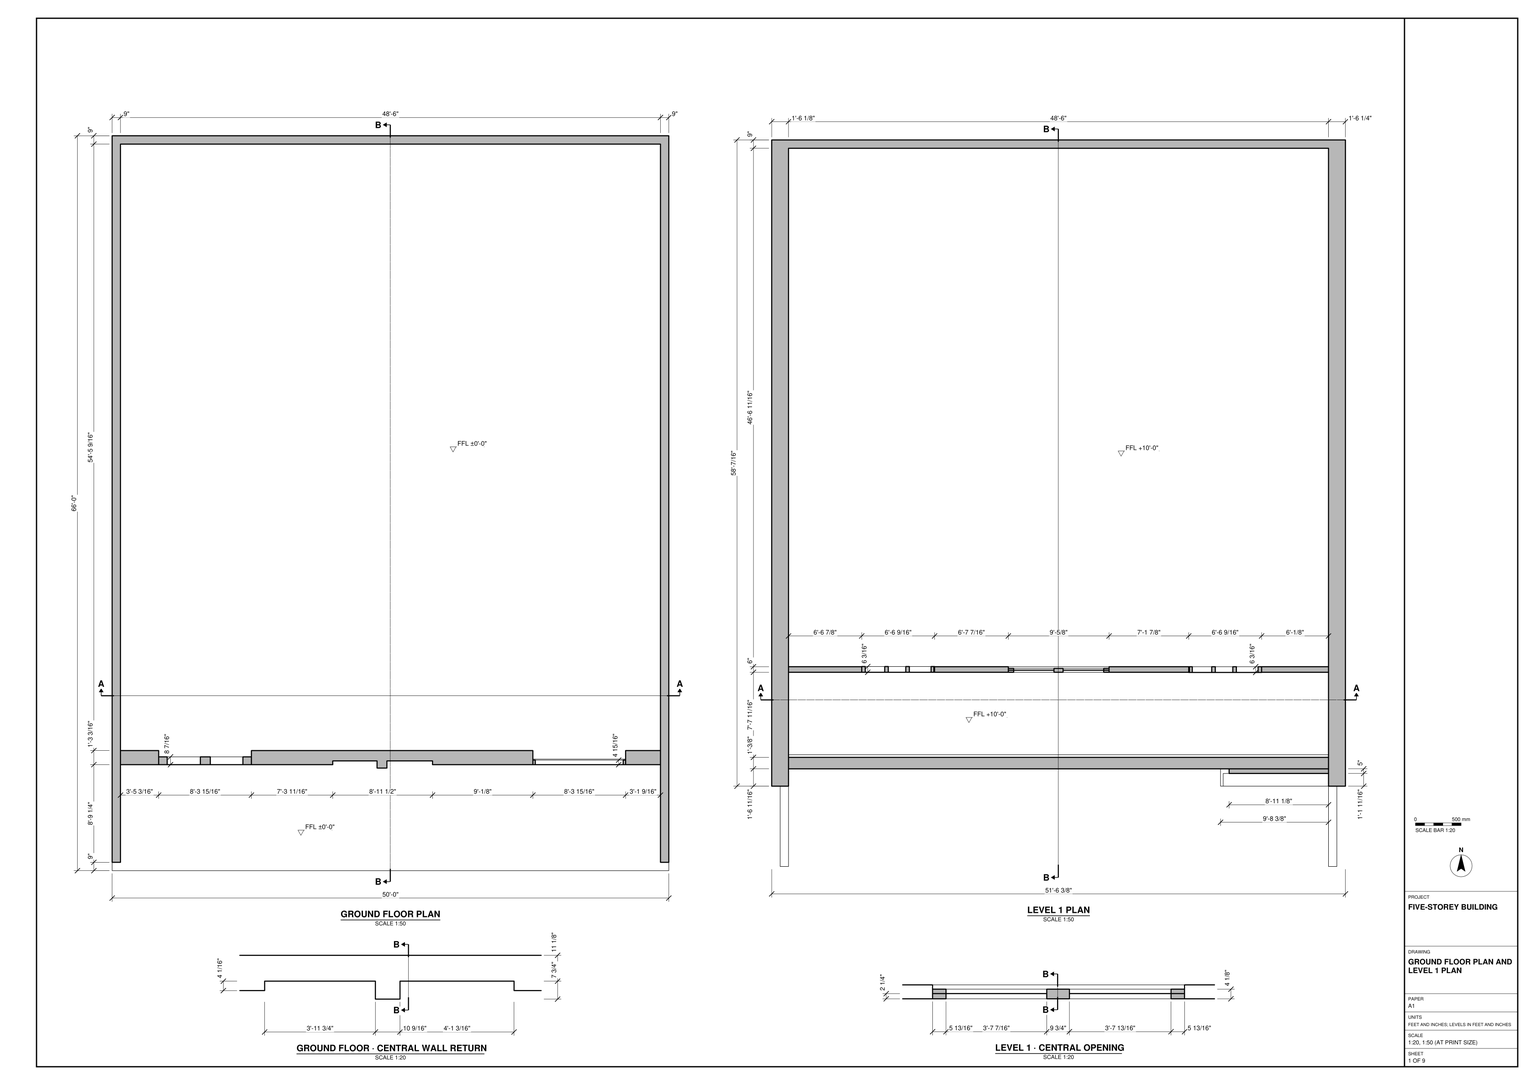
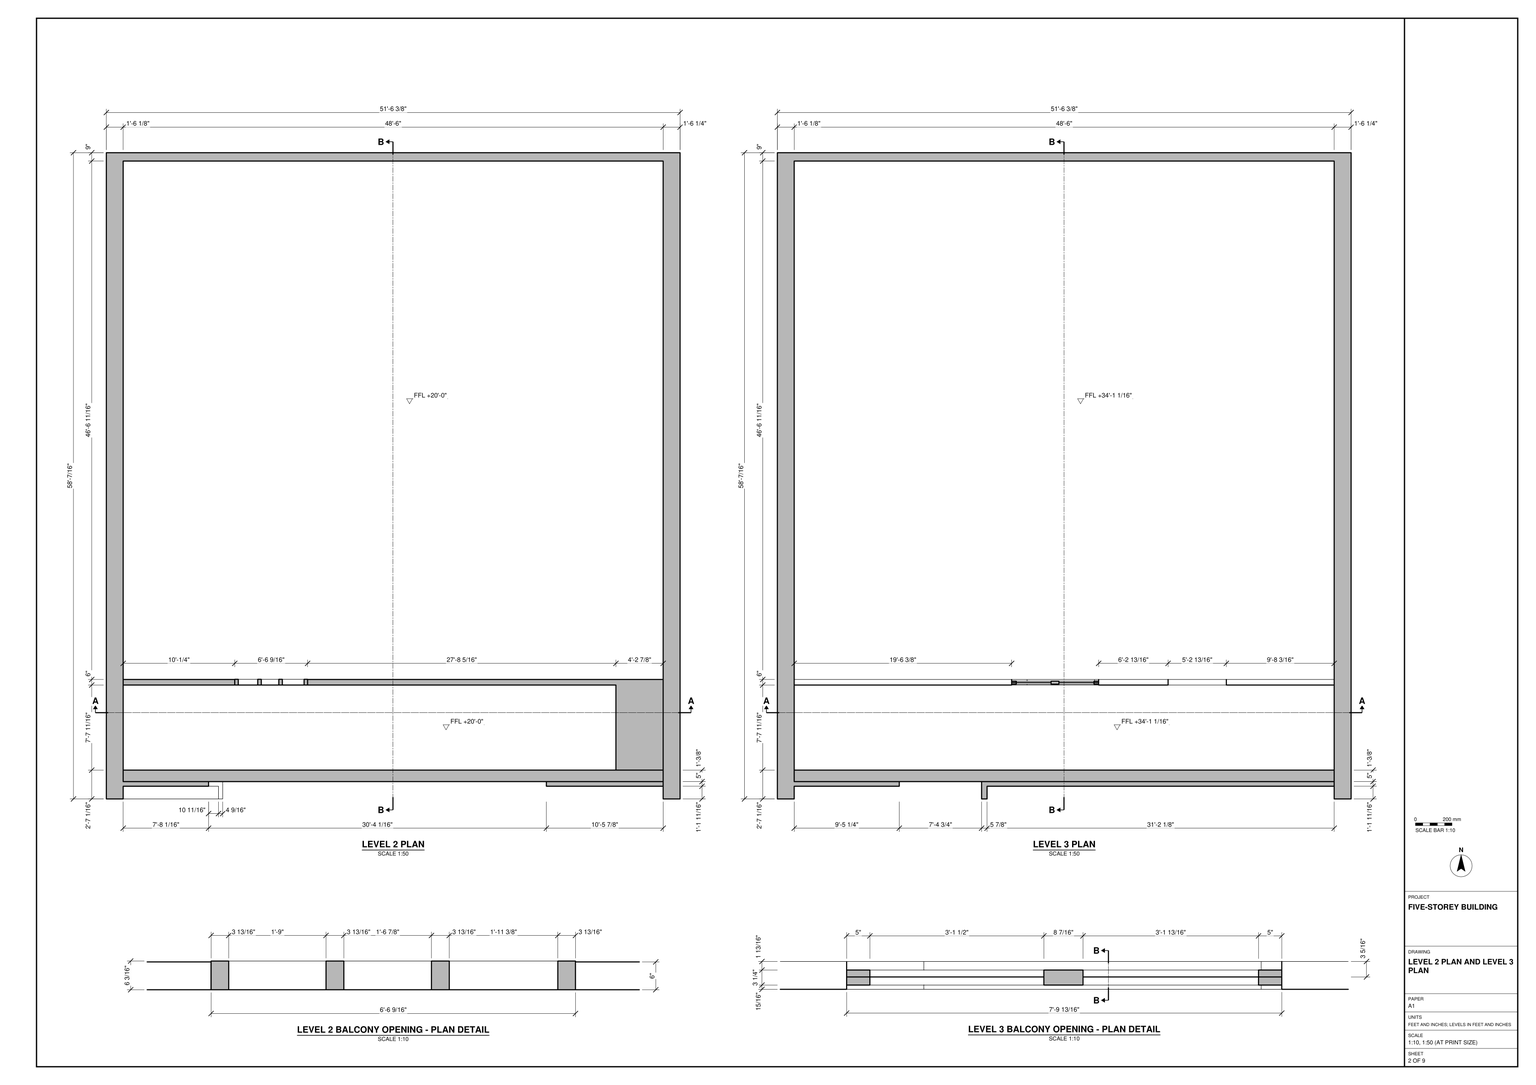
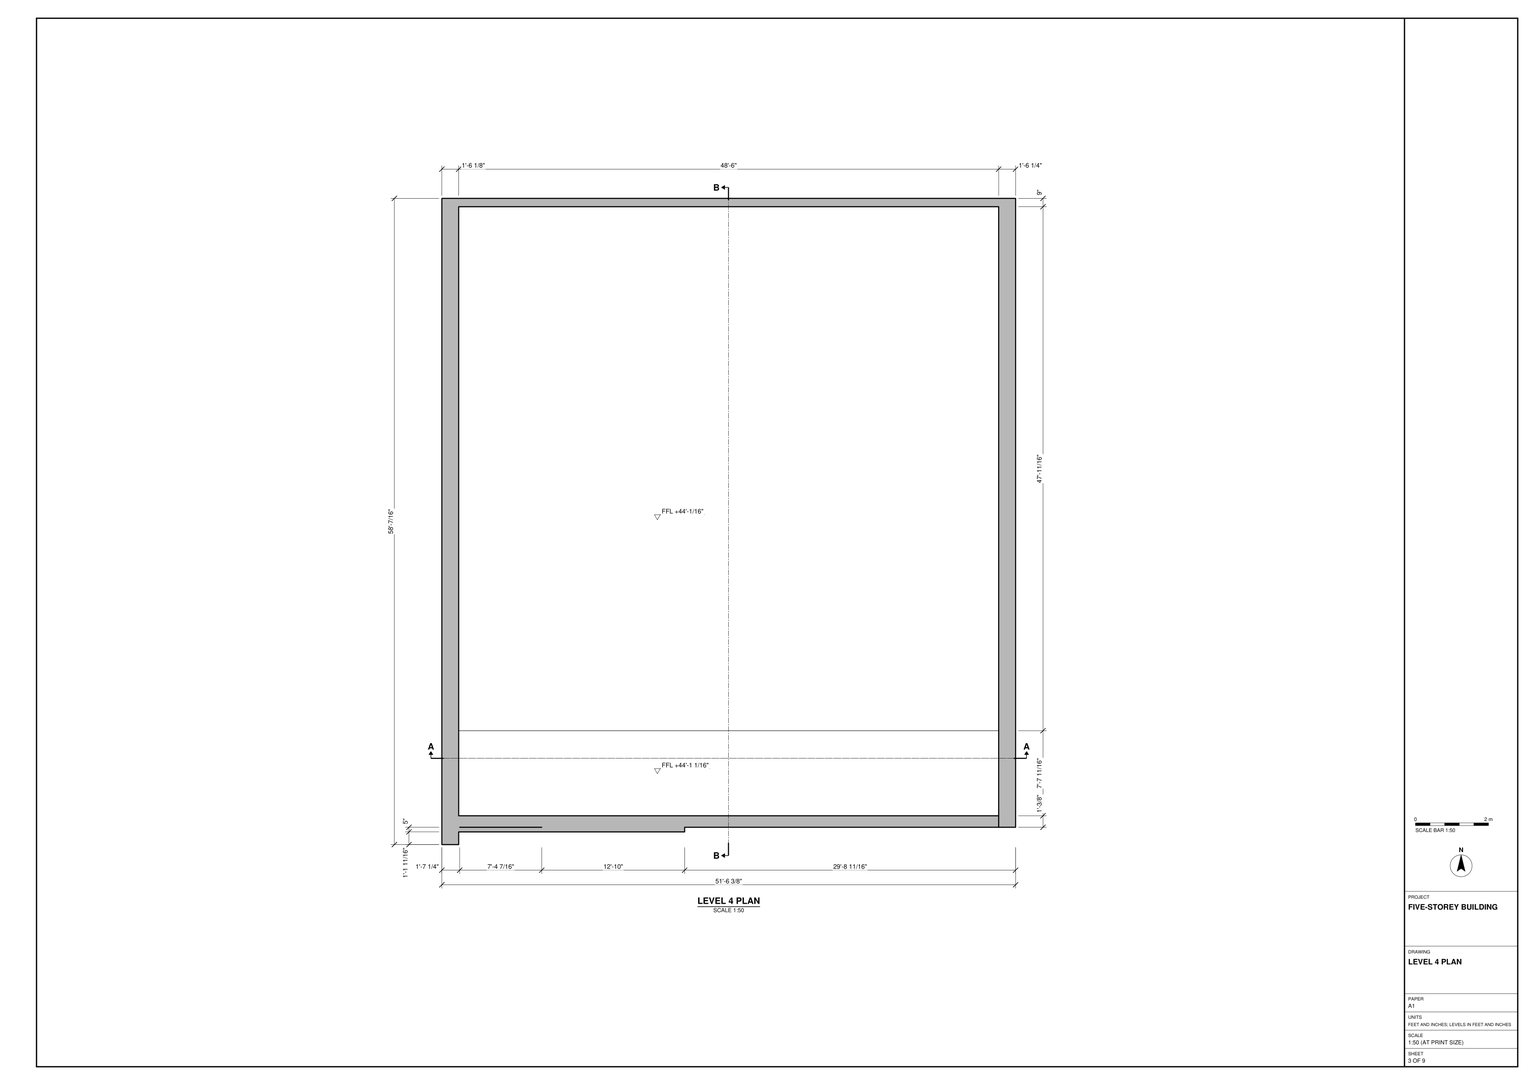
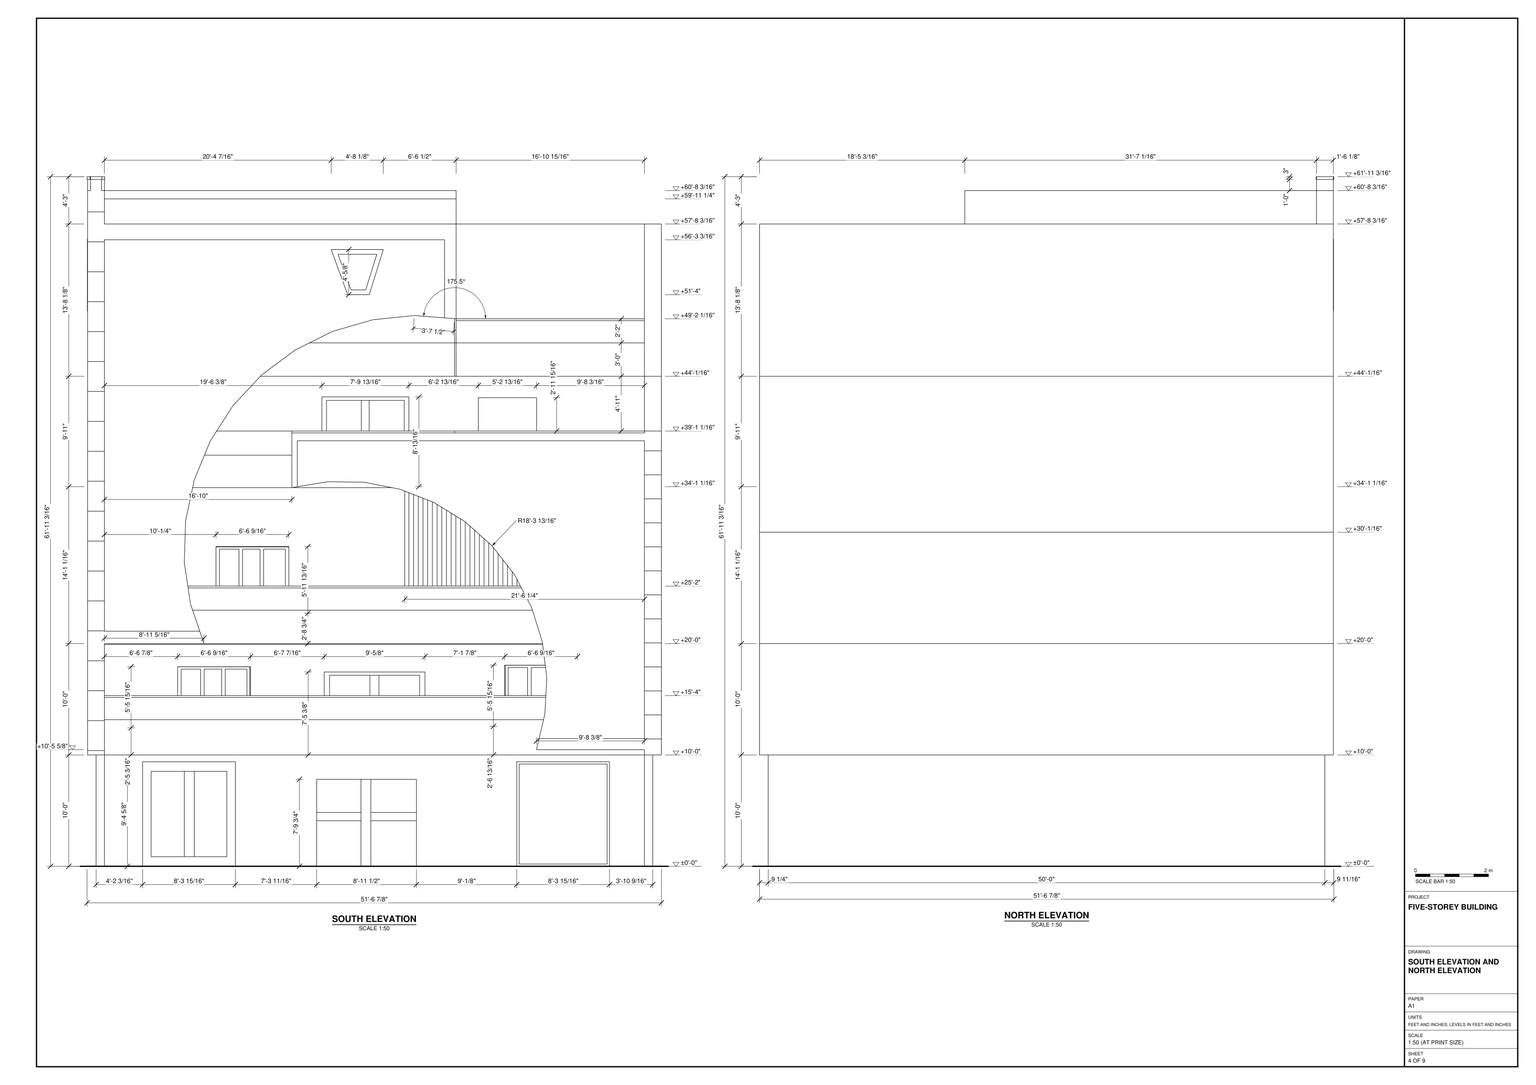
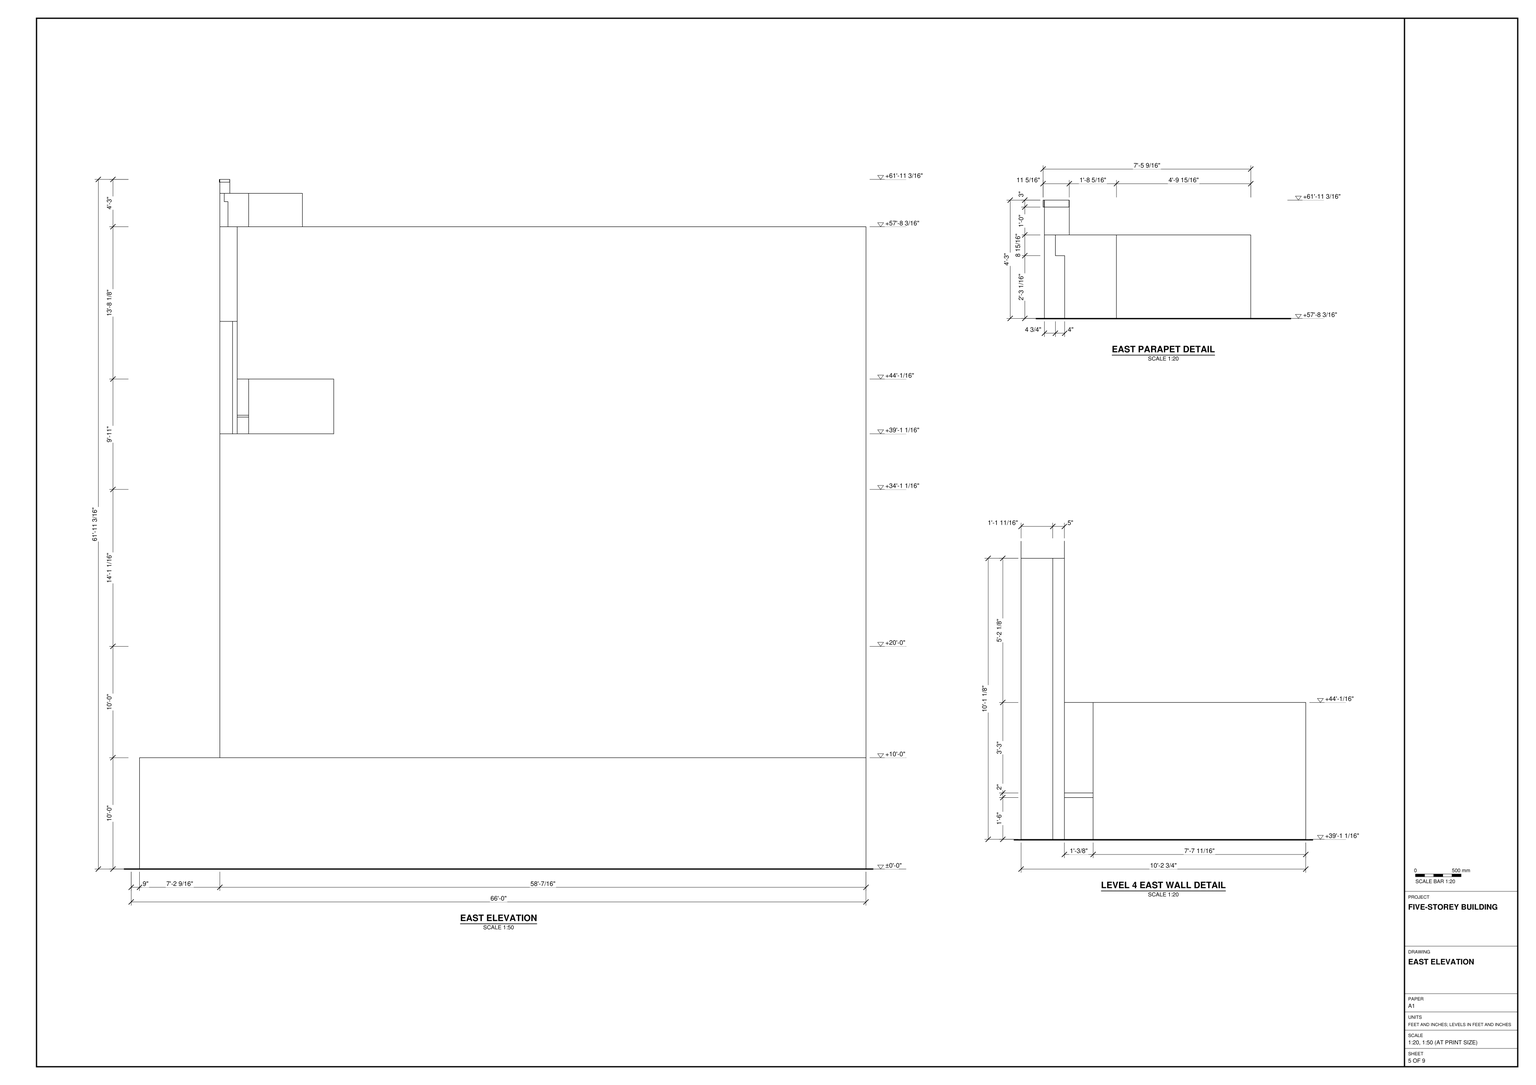
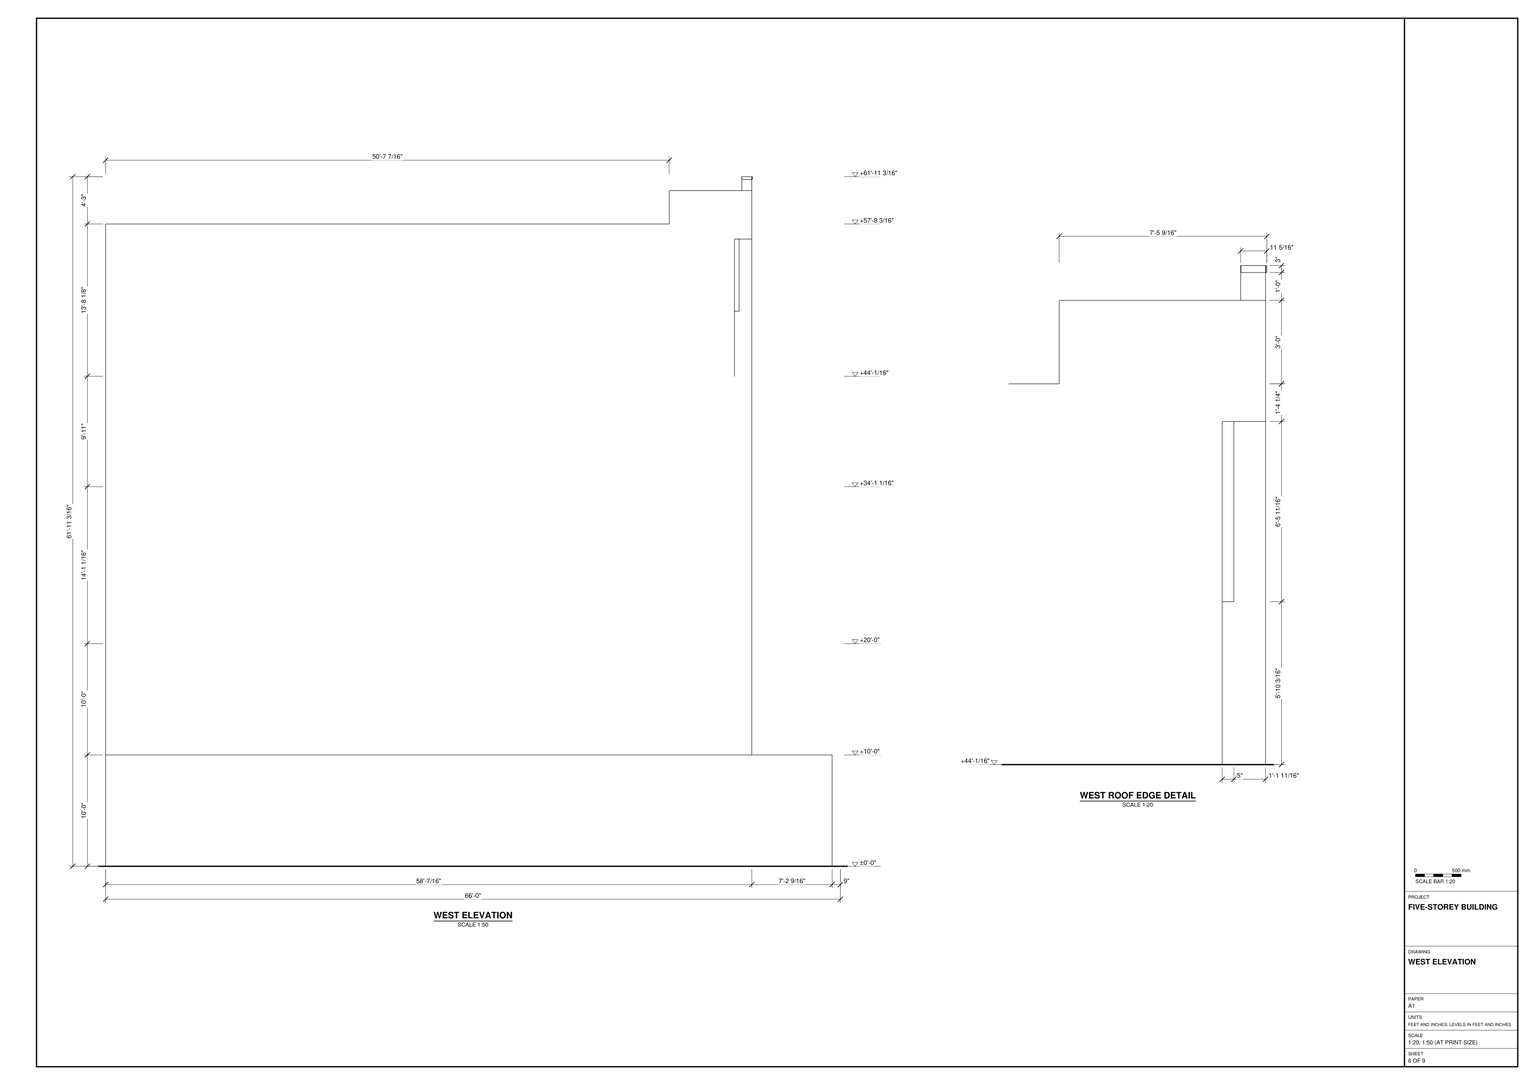
Build the five-storey building in SketchUp from task_files/diagram_01.pdf. Work in feet and inches. The overall width is 51'-6 15/16", the front-to-back depth is 66'-0", and the height is 61'-11 3/16". Set the finished floor levels to ±0'-0", +10'-0", +20'-0", +34'-1 1/16", and +44'-1/16".

Start with the deeper ground-floor slab. Model the side walls extending past the recessed front wall, including the openings on either side of its stepped central return. Use the wall thicknesses drawn at each level: the upper side walls are thicker than those on the ground floor. Keep the large floor areas open as drawn. Form the front balconies on Levels 1 through 3, following each plan for the slab edge, wall returns and framed openings rather than copying one frontage to every level. Follow the Level 4 plan for the stepped front edge and use the sections and elevations to complete the roof and facade above it.

Keep walls, slabs and roof in separate groups or components. Keep each furniture or joinery piece shown separate as well, and use components for repeated parts. Any decor or loose items shown may be represented by suitable library components. Save one SketchUp model as output_files/five_storey_building_with_recessed_front_balconies.skp.

# SketchUp Ruby script. Lengths in inches.
U = 1.inch
M = Sketchup.active_model
def pt(a) = Geom::Point3d.new(a.map { |v| v * U })
def face(e, loops, mat)
  f = e.add_face(loops[0].map { |a| pt(a) })
  loops[1..].each { |l| e.add_face(l.map { |a| pt(a) }).erase! }
  f.material = f.back_material = mat if mat
  f
end
# faces: each face lists its corners as indices into pts; further lists are holes
def faces(e, pts, list, mat = nil) = list.each { |f| face(e, (f[0].is_a?(Array) ? f : [f]).map { |l| l.map { |i| pts[i] } }, mat) }
# xy, xz, yz: faces in a plane at the given z, y or x. An outline is a flat list of corners, or four numbers for a rectangle; further outlines are holes
def ring(l) = l.size == 4 ? [[l[0], l[1]], [l[2], l[1]], [l[2], l[3]], [l[0], l[3]]] : l.each_slice(2).to_a
def flat(e, list, mat, &to3) = list.each { |f| face(e, (f[0].is_a?(Array) ? f : [f]).map { |l| ring(l).map { |u, v| to3.(u, v) } }, mat) }
def xy(e, z, list, mat = nil) = flat(e, list, mat) { |x, y| [x, y, z] }
def xz(e, y, list, mat = nil) = flat(e, list, mat) { |x, z| [x, y, z] }
def yz(e, x, list, mat = nil) = flat(e, list, mat) { |y, z| [x, y, z] }
def lines(e, pts, list) = list.each { |a, b| e.add_line(pt(pts[a]), pt(pts[b])) }
# prism: a flat outline (further loops are holes) pulled along v
def prism(e, loops, v, mat = nil)
  f = face(e, loops, mat); d = Geom::Vector3d.new(v.map { |x| x * U })
  f.pushpull(f.normal.samedirection?(d) ? d.length : -d.length)
end
def box(e, o, s, mat = nil) = prism(e, [[o, [o[0] + s[0], o[1], o[2]], [o[0] + s[0], o[1] + s[1], o[2]], [o[0], o[1] + s[1], o[2]]]], [0, 0, s[2]], mat)
def at(x, y, z, deg = 0) = Geom::Transformation.translation(pt([x, y, z])) * Geom::Transformation.rotation(ORIGIN, Z_AXIS, deg.degrees)
def axes(o, x, y, z) = Geom::Transformation.new([*x, 0, *y, 0, *z, 0, *pt(o).to_a, 1])
def part(name) = M.definitions.add(name)
# library, detail: a bought-in or finely detailed component or shape, given as its bounding box
def library(name, o, s) = part(name).tap { |d| box(d.entities, o, s) }
def detail(e, o, s) = box(e.add_group.entities, o, s)
def put(e, d, t, mat = nil) = e.add_instance(d, t).tap { |i| i.material = mat if mat }
def group(e, t, mat = nil) = e.add_group.tap { |g| g.transformation = t; g.material = mat if mat }.entities
root = M.entities
M.materials.add("[Aluminum]").color = [179, 179, 179]
M.materials.add("[Blinds Roman Hobbled Blue]").color = [81, 82, 87]
M.materials.add("[Blinds Wood Light]").color = [155, 100, 14]
M.materials.add("[Color D06]").color = [204, 153, 0]
M.materials.add("[Color M00]").color = [255, 255, 255]
M.materials.add("[Metal Silver]").color = [234, 233, 238]
M.materials.add("[Polished Concrete Old]").color = [229, 229, 229]
M.materials.add("[Translucent Glass Gray]").color = [128, 128, 128]
M.materials["[Translucent Glass Gray]"].alpha = 0.5
M.materials.add("[Wood Bamboo]").color = [177, 105, 43]
M.materials.add("[Wood Floor]").color = [155, 105, 61]
c1 = part("Group\#3")
xy(c1.entities,0,[[0,0,110.8125,6]])
xy(c1.entities,5.36,[[5.36,0,34.95,6],[40.375,0,67.02,6],[72.4375,0,105.45,6]])
xy(c1.entities,134.51,[[5.36,0,34.95,6],[40.375,0,67.02,6],[72.4375,0,105.45,6]])
xy(c1.entities,139.875,[[0,0,110.8125,6]])
xz(c1.entities,0,[[[0,0,110.8125,139.875],[72.4375,5.36,105.45,134.51],[5.36,5.36,34.95,134.51],[40.375,5.36,67.02,134.51]]])
xz(c1.entities,0,[[5.36,5.36,34.95,134.51],[40.375,5.36,67.02,134.51],[72.4375,5.36,105.45,134.51]],"[Translucent Glass Gray]")
xz(c1.entities,6,[[[0,0,110.8125,139.875],[72.4375,5.36,105.45,134.51],[5.36,5.36,34.95,134.51],[40.375,5.36,67.02,134.51]]])
yz(c1.entities,0,[[0,0,6,139.875]])
yz(c1.entities,5.36,[[0,5.36,6,134.51]])
yz(c1.entities,34.95,[[0,5.36,6,134.51]])
yz(c1.entities,40.375,[[0,5.36,6,134.51]])
yz(c1.entities,67.02,[[0,5.36,6,134.51]])
yz(c1.entities,72.4375,[[0,5.36,6,134.51]])
yz(c1.entities,105.45,[[0,5.36,6,134.51]])
yz(c1.entities,110.8125,[[0,0,6,139.875]])
c2 = part("Group\#4")
xy(c2.entities,0,[[0,0,126.375,7],[0,7,126.375,13]])
xy(c2.entities,6.76,[[57.28,0,68.66,7],[6.76,7,57.28,13],[57.28,7,68.66,13],[68.66,7,119.62,13]])
xy(c2.entities,6.76,[[6.76,0,57.28,7],[68.66,0,119.62,7]],"[Wood Floor]")
xy(c2.entities,165.31,[[57.28,0,68.66,7],[6.76,7,57.28,13],[57.28,7,68.66,13],[68.66,7,119.62,13]])
xy(c2.entities,165.31,[[6.76,0,57.28,7],[68.66,0,119.62,7]],"[Wood Floor]")
xy(c2.entities,172.0625,[[0,0,126.375,7],[0,7,126.375,13]])
xz(c2.entities,0,[[57.28,6.76,68.66,165.31]])
xz(c2.entities,0,[[[0,0,126.375,172.0625],[6.76,6.76,119.62,165.31]]],"[Wood Floor]")
xz(c2.entities,7,[[[0,0,126.375,172.0625],[6.76,6.76,119.62,165.31]]])
xz(c2.entities,7,[[6.76,6.76,57.28,165.31],[68.66,6.76,119.62,165.31]],"[Wood Floor]")
xz(c2.entities,13,[[[0,0,126.375,172.0625],[6.76,6.76,119.62,165.31]],[57.28,6.76,68.66,165.31]])
yz(c2.entities,0,[[0,0,7,172.0625],[7,0,13,172.0625]])
yz(c2.entities,6.76,[[7,6.76,13,165.31]])
yz(c2.entities,6.76,[[0,6.76,7,165.31]],"[Wood Floor]")
yz(c2.entities,57.28,[[0,6.76,7,165.31],[7,6.76,13,165.31]])
yz(c2.entities,68.66,[[0,6.76,7,165.31],[7,6.76,13,165.31]])
yz(c2.entities,119.62,[[7,6.76,13,165.31]])
yz(c2.entities,119.62,[[0,6.76,7,165.31]],"[Wood Floor]")
yz(c2.entities,126.375,[[0,0,7,172.0625],[7,0,13,172.0625]])
xy(root,0,[[9.66,0,609.66,0,609.66,9,600.66,9,600.66,114.25,563.09,114.25,563.09,120.25,463.14,120.25,463.14,114.25,354.98,114.25,354.98,118.3125,305.81,118.3125,305.81,110.5625,295.19,110.5625,295.19,118.3125,247.45,118.3125,247.45,114.25,159.78,114.25,159.78,120.25,59.83,120.25,59.83,114.25,18.66,114.25,18.66,9,9.66,9],[9.66,9,9.66,792,609.66,792,609.66,9,600.66,9,600.66,783,18.66,783,18.66,9],[295.19,110.5625,295.19,118.3125,247.45,118.3125,247.45,114.25,159.78,114.25,159.78,129.4375,463.14,129.4375,463.14,114.25,354.98,114.25,354.98,118.3125,305.81,118.3125,305.81,110.5625],[18.66,114.25,59.83,129.4375],[563.09,114.25,600.66,129.4375],
  [59.83,120.25,159.78,120.25,159.78,129.4375,463.14,129.4375,463.14,120.25,563.09,120.25,563.09,129.4375,600.66,129.4375,600.66,783,18.66,783,18.66,129.4375,59.83,129.4375]])
xy(root,93.73,[[295.19,110.5625,305.81,114.25]])
xy(root,93.73,[[247.45,114.25,295.19,118.3125],[305.81,114.25,354.98,118.3125]],"[Blinds Wood Light]")
xy(root,112.63,[[59.83,114.25,159.78,129.4375],[463.14,114.25,563.09,129.4375]])
xy(root,120,[[9.66,9,18.66,95.5625],[600.66,9,609.66,95.5625],[0.54,95.5625,9.66,792],[609.66,95.5625,618.91,792],[18.66,114.25,600.66,126.625],
  [18.66,126.625,600.66,129.4375],[18.66,129.4375,600.66,129.4375,600.66,218.3125,364.17,218.3125,364.17,224.3125,255.54,224.3125,255.54,218.3125,18.66,218.3125],[18.66,224.3125,600.66,783]])
xy(root,125.65,[[484.29,95.5625,600.66,114.25]],"[Polished Concrete Old]")
xy(root,137.67,[[487.14,95.5625,600.66,109.25]],"[Polished Concrete Old]")
xy(root,149.16,[[97.56,218.3125,175.31,224.3125]])
xy(root,150.8125,[[450.8125,218.3125,528.5625,224.3125]])
xy(root,158,[[18.66,114.25,600.66,126.625]])
xy(root,182,[[18.66,114.25,600.66,126.625]])
xy(root,184,[[18.66,114.25,600.66,126.625]],"[Metal Silver]")
xy(root,209.375,[[255.54,218.3125,364.17,224.3125]])
xy(root,214.97,[[97.56,218.3125,175.31,224.3125]])
xy(root,216.625,[[450.8125,218.3125,528.5625,224.3125]])
xy(root,239,[[18.66,126.625,600.66,218.3125],[18.66,224.3125,600.66,783]])
xy(root,240,[[18.66,95.5625,125.96,114.25],[18.66,114.25,600.66,126.625],[18.66,126.625,549.76,218.3125],[549.76,126.625,600.66,218.3125],[18.66,224.3125,600.66,783]])
xy(root,253.36,[[18.66,95.5625,121.41,109.25]])
xy(root,272.73,[[138.9,218.3125,217.46,224.3125]])
xy(root,276,[[18.66,114.25,600.66,126.625]])
xy(root,300,[[18.66,114.25,600.66,126.625]])
xy(root,302,[[18.66,114.25,600.66,126.625]],"[Metal Silver]")
xy(root,344.17,[[138.9,218.3125,217.46,224.3125]])
xy(root,408.0625,[[18.66,114.25,600.66,126.625],[18.66,126.625,549.76,218.3125],[549.76,126.625,600.66,218.3125],[18.66,218.3125,600.66,224.3125],[18.66,224.3125,600.66,783]])
xy(root,409.0625,[[18.66,126.625,600.66,218.3125],[253.02,218.3125,269.66,224.3125],[269.66,218.3125,342.38,224.3125],[342.38,218.3125,346.82,224.3125],[18.66,224.3125,600.66,783]])
xy(root,442.21,[[421.65,218.3125,484.46,224.3125]])
xy(root,443.0625,[[18.66,114.25,600.66,126.625]])
xy(root,458.58,[[226.55,95.5625,600.66,109.25]],"[Polished Concrete Old]")
xy(root,467.0625,[[220.66,95.5625,600.66,109.25],[220.66,109.25,600.66,114.25]],"[Polished Concrete Old]")
xy(root,469.0625,[[600.66,95.5625,618.91,218.3125]])
xy(root,469.0625,[[18.66,114.25,600.66,126.625]],"[Metal Silver]")
xy(root,505.02,[[421.65,218.3125,484.46,224.3125]])
xy(root,505.86,[[253.02,218.3125,346.82,224.3125]])
xy(root,528.0625,[[18.66,114.25,600.66,126.625],[18.66,126.625,600.66,218.3125],[18.66,218.3125,600.66,783]])
xy(root,528.0625,[[600.66,114.25,618.91,218.3125]],"[Polished Concrete Old]")
xy(root,529.0625,[[18.66,126.625,600.66,218.3125]])
xy(root,564.0625,[[18.66,114.25,600.66,126.625]])
xy(root,590.0625,[[397.73,114.25,397.75,126.625],[397.75,114.25,600.66,126.625]],"[Metal Silver]")
xy(root,590.19,[[396.08,95.5625,397.73,114.25]])
xy(root,598.28,[[0.27,109.25,0.54,114.25]])
xy(root,616.02,[[280.84,95.5625,304.09,109.25]],"[Color M00]")
xy(root,621.15,[[284.43,95.5625,300.3125,109.25]],"[Color M00]")
xy(root,659.53,[[270.42,95.5625,312.24,109.25]],"[Color M00]")
xy(root,664.66,[[263.09,95.5625,319.21,109.25]],"[Color M00]")
xy(root,675.1875,[[18.66,95.5625,385.27,109.25]])
xy(root,675.97,[[0.27,109.25,0.54,114.25]])
xy(root,692.1875,[[18.66,95.5625,397.73,104.3125],[600.66,114.25,618.91,114.25,618.91,792,0.54,792,0.54,184.54,18.66,184.54,18.66,783,600.66,783]])
xy(root,719.25,[[18.66,100.3125,397.73,104.3125]],"[Color M00]")
xy(root,728.1875,[[0.54,95.5625,3.7,95.5625,0.54,106.31],[15.52,95.5625,18.66,95.5625,18.66,106.31],[18.66,100.3125,397.73,126.625],[0.54,106.31,18.66,184.54]])
xy(root,740.1875,[[3.2,95,3.2,95.42,3.7,95.5625,3.7,95],[3.7,95,3.7,95.5625,15.52,95.5625,15.94,95.44,15.96,95.5,15.96,95],[3.16,95.4,0,106.15,0.54,106.31,3.7,95.5625,3.2,95.5625,3.2,95.42],[3.2,95.42,3.2,95.5625,3.7,95.5625],[15.94,95.44,15.52,95.5625,15.96,95.5625,15.96,95.5],
  [15.96,95.5,15.96,95.5625,15.52,95.5625,18.66,106.31,19.08,106.18],[[3.7,95.5625,0.54,106.31,18.66,106.31,15.52,95.5625],[4.6875,96.88,14.54,96.88,16.9,104.99,2.3,104.99]],[4.6875,96.88,14.54,96.88,16.9,104.99,2.3,104.99]])
xy(root,743.1875,[[3.2,95,3.7,95,3.7,95.5625,0.54,106.31,0,106.15,3.16,95.4,3.2,95.42],[[3.7,95,15.96,95,15.96,95.5,19.08,106.18,18.66,106.31,0.54,106.31,3.7,95.5625],[4.6875,96.88,2.3,104.99,16.9,104.99,14.54,96.88]]])
xz(root,9,[[9.66,0,18.66,120],[600.66,0,609.66,120]])
xz(root,95,[[3.2,740.1875,3.7,743.1875],[3.7,740.1875,15.96,743.1875]])
xz(root,95.5625,[[0.54,120,18.66,124.73],[600.66,120,618.91,120,618.91,163.13,600.66,163.13,600.66,137.67,487.14,137.67,484.29,125.65,600.66,125.65],[0.54,124.73,18.66,156.98],[0.54,156.98,18.66,189.23],[600.66,163.13,618.91,189],
  [600.66,189,618.91,214.88],[0.54,189.23,18.66,221.48],[600.66,214.88,618.91,240.75],[0.54,221.48,18.66,221.48,18.66,240,125.96,240,121.41,253.36,18.66,253.36,18.66,253.73,0.54,253.73],[600.66,240.75,618.91,266.63],
  [0.54,253.73,18.66,285.98],[600.66,266.63,618.91,292.5],[0.54,285.98,18.66,318.23],[600.66,292.5,618.91,318.38],[0.54,318.23,18.66,350.48],
  [600.66,318.38,618.91,344.25],[600.66,344.25,618.91,370.13],[0.54,350.48,18.66,382.73],[600.66,370.13,618.91,396],[0.54,382.73,18.66,414.98],
  [600.66,396,618.91,421.88],[220.66,408.0625,226.55,409.04,226.55,458.58,600.66,458.58,600.66,447.75,618.91,447.75,618.91,469.0625,600.66,469.0625,600.66,467.0625,220.66,467.0625],[0.54,414.98,18.66,447.23],[600.66,421.88,618.91,447.75],[0.54,447.23,18.66,479.48],
  [0.54,479.48,18.66,511.73],[0.54,511.73,18.66,543.98],[0.54,543.98,18.66,576.23],[0.54,576.23,18.66,608.48],[396.08,590.19,397.73,590.19,397.73,692.1875,18.66,692.1875,18.66,705.23,0.54,705.23,0.54,672.98,18.66,672.98,18.66,675.1875,385.27,675.1875,385.27,591.03],
  [0.54,608.48,18.66,640.73],[0.54,640.73,18.66,672.98],[0.54,705.23,18.66,705.23,18.66,728.1875,15.52,728.1875,15.52,740.1875,3.7,740.1875,3.7,728.1875,0.54,728.1875]])
xz(root,95.5625,[[[280.84,616.02,304.09,616.02,319.21,664.66,263.09,664.66],[284.43,621.15,270.42,659.53,312.24,659.53,300.3125,621.15]]],"[Color M00]")
xz(root,96.88,[[4.6875,740.1875,14.54,743.1875]])
xz(root,100.3125,[[18.66,719.25,397.73,728.1875]],"[Color M00]")
xz(root,104.3125,[[18.66,692.1875,397.73,719.25]],"[Color M00]")
xz(root,104.99,[[2.3,740.1875,16.9,743.1875]])
xz(root,106.31,[[0.54,728.1875,18.66,740.1875],[0.54,740.1875,18.66,743.1875]])
xz(root,109.25,[[0.27,598.28,0.54,675.97]])
xz(root,109.25,[[284.43,621.15,300.3125,621.15,312.24,659.53,270.42,659.53]],"[Color M00]")
xz(root,109.25,[[487.14,137.67,600.66,137.67,600.66,458.58,226.55,458.58,226.55,409.04,259.41,414.48,298.67,413.91,337.21,406.35,373.79,392.0625,407.24,371.49,436.5,345.29,460.62,314.3,478.85,279.52,490.59,242.04,495.48,203.08,493.36,163.86],[[18.66,253.36,121.41,253.36,111.41,282.72,104.73,327.36,106.14,372.47,115.59,416.6,132.77,458.33,157.13,496.32,187.9,529.34,224.07,556.34,264.48,576.43,307.83,588.97,352.73,593.57,385.27,591.03,385.27,675.1875,18.66,675.1875],[280.84,616.02,263.09,664.66,319.21,664.66,304.09,616.02]]],"[Wood Bamboo]")
xz(root,110.5625,[[295.19,0,305.81,93.73]])
xz(root,114.25,[[18.66,0,59.83,0,59.83,112.63,159.78,112.63,159.78,0,247.45,0,247.45,93.73,354.98,93.73,354.98,0,463.14,0,463.14,112.63,563.09,112.63,563.09,0,600.66,0,600.66,120,18.66,120],[18.66,240,19.77,276],[19.77,240,108.21,276],[108.21,240,108.21,276,113.7,276,125.96,240],[490.85,240,490.59,242.04,479.95,276,600.66,276,600.66,240],
  [18.66,276,18.66,564.0625,19.77,564.0625,19.77,598.28,108.21,598.28,108.21,528.0625,19.77,528.0625,19.77,469.0625,108.21,469.0625,108.21,467.0625,19.77,467.0625,19.77,302,108.21,302,108.21,276],[18.66,276,19.77,300],[108.21,276,108.21,300,108.83,300,111.41,282.72,113.7,276],[18.66,302,19.77,408.0625],[19.77,302,19.77,408.0625,113.76,408.0625,106.14,372.47,104.73,327.36,108.53,302],
  [19.77,443.0625,19.77,467.0625,138.37,467.0625,132.77,458.33,126.48,443.0625],[220.66,443.0625,600.66,467.0625],[220.66,467.0625,396.08,469.0625],[396.08,467.0625,600.66,469.0625],[18.66,469.0625,19.77,528.0625],
  [108.21,528.0625,108.21,564.0625,239.61,564.0625,224.07,556.34,187.9,529.34,186.7,528.0625],[186.7,528.0625,396.08,528.0625,396.08,564.0625,239.61,564.0625,224.07,556.34,187.9,529.34],[19.77,564.0625,108.21,598.28],[239.61,564.0625,396.08,564.0625,396.08,590.19,352.73,593.57,307.83,588.97,264.48,576.43],[396.08,564.0625,397.75,564.0625,397.75,590.0625,397.73,590.0625,397.73,590.19,396.08,590.19],
  [0.27,598.28,0.54,675.97]])
xz(root,114.25,[[18.66,182,494.34,182,494.45,184,18.66,184],[18.66,300,19.77,302],[19.77,300,108.21,302],[108.21,300,108.21,302,108.53,302,108.83,300],[108.83,300,108.53,302,467.07,302,468.12,300],
  [468.12,300,600.66,300,600.66,302,467.07,302],[18.66,467.0625,19.77,469.0625],[19.77,467.0625,108.21,469.0625],[108.21,467.0625,108.21,469.0625,139.65,469.0625,138.37,467.0625],[397.75,588.0625,600.66,590.0625]],"[Metal Silver]")
xz(root,114.25,[[18.66,120,18.66,158,491.97,158,484.29,125.65,600.66,125.65,600.66,120],[484.29,125.65,491.97,158,600.66,158,600.66,125.65],[494.45,184,495.48,203.08,490.85,240,600.66,240,600.66,184],[125.96,240,490.85,240,490.59,242.04,479.95,276,113.7,276],[467.07,302,460.62,314.3,436.5,345.29,407.24,371.49,373.79,392.0625,337.21,406.35,328.5,408.0625,600.66,408.0625,600.66,302],
  [18.66,408.0625,19.77,443.0625],[19.77,408.0625,19.77,443.0625,126.48,443.0625,115.59,416.6,113.76,408.0625],[113.76,408.0625,115.59,416.6,126.48,443.0625,220.66,443.0625,220.66,408.0625],[220.66,408.0625,259.41,414.48,298.67,413.91,328.5,408.0625,600.66,408.0625,600.66,443.0625,220.66,443.0625],[220.66,408.0625,328.5,408.0625,298.67,413.91,259.41,414.48],
  [18.66,528.0625,19.77,564.0625],[19.77,528.0625,108.21,564.0625],[396.08,528.0625,397.75,564.0625],[397.75,528.0625,600.66,564.0625],[600.66,528.0625,618.91,692.1875]],"[Polished Concrete Old]")
xz(root,114.25,[[18.66,158,491.97,158,493.36,163.86,494.34,182,18.66,182],[491.97,158,493.36,163.86,494.34,182,600.66,182,600.66,158],[19.77,276,108.21,300],[113.7,276,479.95,276,478.85,279.52,468.12,300,108.83,300,111.41,282.72],[479.95,276,478.85,279.52,468.12,300,600.66,300,600.66,276],
  [18.66,443.0625,19.77,467.0625],[126.48,443.0625,220.66,443.0625,220.66,469.0625,139.65,469.0625,138.37,467.0625,132.77,458.33],[397.75,564.0625,600.66,588.0625]],"[Translucent Glass Gray]")
xz(root,118.3125,[[247.45,49.12,295.19,58],[305.81,49.12,354.98,58]],"[Blinds Roman Hobbled Blue]")
xz(root,118.3125,[[247.45,0,295.19,49.12],[305.81,0,354.98,49.12],[247.45,58,295.19,93.73],[305.81,58,354.98,93.73]],"[Blinds Wood Light]")
xz(root,126.625,[[18.66,120,600.66,158],[18.66,239,600.66,240],[18.66,240,549.76,276],[549.76,240,600.66,276],[549.76,302,600.66,408.0625],
  [18.66,408.0625,600.66,409.0625],[220.66,409.0625,600.66,443.0625],[220.66,443.0625,600.66,467.0625],[220.66,467.0625,600.66,469.0625],[18.66,528.0625,600.66,529.0625],
  [18.66,529.0625,600.66,564.0625],[18.66,564.0625,397.75,588.0625],[18.66,590.0625,397.73,692.1875],[18.66,692.1875,397.73,728.1875]])
xz(root,126.625,[[18.66,182,600.66,184],[18.66,300,549.76,302],[549.76,300,600.66,302],[18.66,467.0625,220.66,469.0625],[18.66,588.0625,397.75,590.0625],
  [397.75,588.0625,600.66,590.0625]],"[Metal Silver]")
xz(root,126.625,[[18.66,409.0625,220.66,443.0625]],"[Polished Concrete Old]")
xz(root,126.625,[[18.66,158,600.66,182],[18.66,276,549.76,300],[549.76,276,600.66,300],[18.66,443.0625,220.66,467.0625],[397.75,564.0625,600.66,588.0625]],"[Translucent Glass Gray]")
xz(root,129.4375,[[18.66,0,18.66,120,600.66,120,600.66,0,563.09,0,563.09,112.63,463.14,112.63,463.14,0,159.78,0,159.78,112.63,59.83,112.63,59.83,0]])
xz(root,184.54,[[0.54,692.1875,18.66,728.1875]])
xz(root,218.3125,[[[18.66,120,255.54,120,255.54,209.375,364.17,209.375,364.17,120,600.66,120,600.66,239,18.66,239],[97.56,149.16,175.31,214.97],[450.8125,150.8125,528.5625,216.625]],[18.66,239,342.38,240],[342.38,239,600.66,240],[[18.66,240,342.38,408.0625],[138.9,272.73,217.46,344.17]],[18.66,408.0625,269.66,409.0625],
  [269.66,408.0625,342.38,409.0625],[342.38,408.0625,346.82,409.0625],[346.82,408.0625,351.88,409.0625],[351.88,408.0625,356.95,409.0625],[356.95,408.0625,362.01,409.0625],
  [362.01,408.0625,367.07,409.0625],[367.07,408.0625,372.13,409.0625],[372.13,408.0625,377.2,409.0625],[377.2,408.0625,382.26,409.0625],[382.26,408.0625,387.32,409.0625],
  [387.32,408.0625,392.38,409.0625],[392.38,408.0625,397.45,409.0625],[397.45,408.0625,402.51,409.0625],[402.51,408.0625,407.57,409.0625],[407.57,408.0625,412.63,409.0625],
  [412.63,408.0625,417.7,409.0625],[417.7,408.0625,422.76,409.0625],[422.76,408.0625,427.82,409.0625],[427.82,408.0625,432.88,409.0625],[432.88,408.0625,437.95,409.0625],
  [437.95,408.0625,443.01,409.0625],[443.01,408.0625,448.07,409.0625],[448.07,408.0625,453.13,409.0625],[453.13,408.0625,458.2,409.0625],[458.2,408.0625,463.26,409.0625],
  [463.26,408.0625,468.32,409.0625],[468.32,408.0625,473.38,409.0625],[473.38,408.0625,478.2,409.0625],[478.2,408.0625,483.01,409.0625],[483.01,408.0625,487.82,409.0625],
  [487.82,408.0625,492.63,409.0625],[492.63,408.0625,497.45,409.0625],[497.45,408.0625,502.26,409.0625],[502.26,408.0625,507.07,409.0625],[507.07,408.0625,511.88,409.0625],
  [511.88,408.0625,516.7,409.0625],[516.7,408.0625,521.51,409.0625],[521.51,408.0625,526.32,409.0625],[526.32,408.0625,531.13,409.0625],[531.13,408.0625,535.95,409.0625],
  [535.95,408.0625,540.76,409.0625],[540.76,408.0625,545.57,409.0625],[545.57,408.0625,549.76,409.0625],[549.76,408.0625,600.66,409.0625],[[18.66,409.0625,253.02,409.0625,253.02,505.86,346.82,505.86,346.82,409.0625,600.66,409.0625,600.66,528.0625,18.66,528.0625],[421.65,442.21,484.46,505.02]],
  [18.66,528.0625,600.66,529.0625]])
xz(root,218.3125,[[342.38,240,346.82,408.0625],[346.82,240,351.88,408.0625],[351.88,240,356.95,408.0625],[356.95,240,362.01,408.0625],[362.01,240,367.07,408.0625],
  [367.07,240,372.13,408.0625],[372.13,240,377.2,408.0625],[377.2,240,382.26,408.0625],[382.26,240,387.32,408.0625],[387.32,240,392.38,408.0625],
  [392.38,240,397.45,408.0625],[397.45,240,402.51,408.0625],[402.51,240,407.57,408.0625],[407.57,240,412.63,408.0625],[412.63,240,417.7,408.0625],
  [417.7,240,422.76,408.0625],[422.76,240,427.82,408.0625],[427.82,240,432.88,408.0625],[432.88,240,437.95,408.0625],[437.95,240,443.01,408.0625],
  [443.01,240,448.07,408.0625],[448.07,240,453.13,408.0625],[453.13,240,458.2,408.0625],[458.2,240,463.26,408.0625],[463.26,240,468.32,408.0625],
  [468.32,240,473.38,408.0625],[473.38,240,478.2,408.0625],[478.2,240,483.01,408.0625],[483.01,240,487.82,408.0625],[487.82,240,492.63,408.0625],
  [492.63,240,497.45,408.0625],[497.45,240,502.26,408.0625],[502.26,240,507.07,408.0625],[507.07,240,511.88,408.0625],[511.88,240,516.7,408.0625],
  [516.7,240,521.51,408.0625],[521.51,240,526.32,408.0625],[526.32,240,531.13,408.0625],[531.13,240,535.95,408.0625],[535.95,240,540.76,408.0625],
  [540.76,240,545.57,408.0625],[545.57,240,549.76,408.0625]],"[Color D06]")
xz(root,218.3125,[[600.66,469.0625,618.91,528.0625]],"[Polished Concrete Old]")
xz(root,224.3125,[[[18.66,120,18.66,239,600.66,239,600.66,120,364.17,120,364.17,209.375,255.54,209.375,255.54,120],[97.56,149.16,175.31,214.97],[450.8125,150.8125,528.5625,216.625]],[18.66,239,600.66,240],[[18.66,240,600.66,408.0625],[138.9,272.73,217.46,344.17]],[18.66,408.0625,552.66,409.0625],[552.66,408.0625,600.66,409.0625]])
xz(root,783,[[18.66,0,600.66,120],[18.66,120,600.66,239],[18.66,239,50.29,240],[50.29,239,600.66,240],[18.66,240,600.66,408.0625],
  [18.66,408.0625,600.66,409.0625],[18.66,409.0625,600.66,528.0625],[18.66,528.0625,600.66,529.0625],[18.66,529.0625,600.66,692.1875]])
xz(root,792,[[9.66,0,609.66,120],[0.54,120,618.91,240],[0.54,240,618.91,360.0625],[0.54,360.0625,618.91,528.0625],[0.54,528.0625,618.91,692.1875]])
yz(root,0.27,[[109.25,598.28,114.25,675.97]])
yz(root,0.54,[[95.5625,120,95.5625,675.97,109.25,675.97,109.25,598.28,114.25,598.28,114.25,675.97,95.5625,675.97,95.5625,728.1875,184.54,728.1875,184.54,692.1875,792,692.1875,792,120],[109.25,598.28,114.25,675.97]])
yz(root,3.2,[[95,740.1875,95.5625,743.1875]])
yz(root,3.7,[[95,740.1875,95.5625,743.1875]])
yz(root,9.66,[[9,0,792,120]])
yz(root,15.96,[[95,740.1875,95.5625,743.1875]])
yz(root,18.66,[[9,0,114.25,120],[114.25,0,129.4375,120],[129.4375,0,783,120],[95.5625,120,114.25,120,114.25,184,126.625,184,126.625,120,218.3125,120,218.3125,239,126.625,239,126.625,240,95.5625,240],[114.25,120,126.625,158],
  [218.3125,120,224.3125,240],[224.3125,120,783,239],[114.25,158,126.625,168],[114.25,168,126.625,182],[114.25,182,126.625,184],
  [126.625,239,218.3125,240],[224.3125,239,783,240],[114.25,240,126.625,276],[126.625,240,218.3125,408.0625],[218.3125,240,224.3125,360.0625],
  [224.3125,240,783,408.0625],[95.5625,253.36,109.25,675.1875],[114.25,276,126.625,300],[114.25,300,126.625,302],[114.25,302,126.625,360.0625],
  [114.25,360.0625,126.625,408.0625],[218.3125,360.0625,224.3125,408.0625],[114.25,408.0625,126.625,443.0625],[126.625,408.0625,218.3125,409.0625],[218.3125,408.0625,224.3125,528.0625],
  [224.3125,408.0625,783,409.0625],[126.625,409.0625,218.3125,528.0625],[224.3125,409.0625,783,528.0625],[114.25,443.0625,126.625,467.0625],[114.25,467.0625,126.625,469.0625],
  [114.25,469.0625,126.625,487.0625],[114.25,489.0625,126.625,528.0625],[126.625,528.0625,218.3125,529.0625],[218.3125,528.0625,224.3125,528.0625,224.3125,529.0625,783,529.0625,783,692.1875,126.625,692.1875,126.625,529.0625,218.3125,529.0625],[224.3125,528.0625,241.3125,529.0625],
  [241.3125,528.0625,783,529.0625],[95.5625,692.1875,104.3125,692.1875,104.3125,719.25,100.3125,719.25,100.3125,728.1875,95.5625,728.1875],[126.625,692.1875,184.54,728.1875]])
yz(root,18.66,[[114.25,487.0625,126.625,489.0625]],"[Aluminum]")
yz(root,59.83,[[114.25,0,129.4375,112.63]])
yz(root,97.56,[[218.3125,149.16,224.3125,214.97]])
yz(root,138.9,[[218.3125,272.73,224.3125,344.17]])
yz(root,159.78,[[114.25,0,129.4375,112.63]])
yz(root,175.31,[[218.3125,149.16,224.3125,214.97]])
yz(root,217.46,[[218.3125,272.73,224.3125,344.17]])
yz(root,220.66,[[95.5625,408.0625,114.25,467.0625]],"[Polished Concrete Old]")
yz(root,226.55,[[95.5625,409.04,109.25,458.58]],"[Polished Concrete Old]")
yz(root,247.45,[[114.25,49.12,118.3125,58]],"[Blinds Roman Hobbled Blue]")
yz(root,247.45,[[114.25,0,118.3125,49.12],[114.25,58,118.3125,93.73]],"[Blinds Wood Light]")
yz(root,253.02,[[218.3125,409.0625,224.3125,505.86]])
yz(root,255.54,[[218.3125,120,224.3125,209.375]])
yz(root,295.19,[[110.5625,0,118.3125,93.73]])
yz(root,305.81,[[110.5625,0,118.3125,93.73]])
yz(root,346.82,[[218.3125,409.0625,224.3125,505.86]])
yz(root,354.98,[[114.25,49.12,118.3125,58]],"[Blinds Roman Hobbled Blue]")
yz(root,354.98,[[114.25,0,118.3125,49.12],[114.25,58,118.3125,93.73]],"[Blinds Wood Light]")
yz(root,364.17,[[218.3125,120,224.3125,209.375]])
yz(root,385.27,[[95.5625,591.03,109.25,675.1875]])
yz(root,397.73,[[114.25,590.0625,126.625,590.0625,126.625,692.1875,95.5625,692.1875,95.5625,590.19,114.25,590.19],[104.3125,692.1875,126.625,692.1875,126.625,728.1875,100.3125,728.1875,100.3125,719.25,104.3125,719.25]])
yz(root,421.65,[[218.3125,442.21,224.3125,505.02]])
yz(root,450.8125,[[218.3125,150.8125,224.3125,216.625]])
yz(root,463.14,[[114.25,0,129.4375,112.63]])
yz(root,484.46,[[218.3125,442.21,224.3125,505.02]])
yz(root,528.5625,[[218.3125,150.8125,224.3125,216.625]])
yz(root,549.76,[[126.625,240,218.3125,408.0625]])
yz(root,563.09,[[114.25,0,129.4375,112.63]])
yz(root,600.66,[[9,0,9,120,95.5625,120,95.5625,125.65,114.25,125.65,114.25,0],[114.25,0,129.4375,120],[129.4375,0,783,120],[114.25,120,126.625,158],[126.625,120,126.625,184,114.25,184,114.25,240,126.625,240,126.625,239,218.3125,239,218.3125,120],
  [218.3125,120,224.3125,240],[224.3125,120,783,239],[95.5625,137.67,109.25,458.58],[114.25,158,126.625,168],[109.25,168,114.25,182],
  [114.25,168,126.625,182],[109.25,182,126.625,184],[126.625,239,218.3125,240],[224.3125,239,783,240],[109.25,240,114.25,276],
  [126.625,240,224.3125,360.0625],[224.3125,240,783,408.0625],[109.25,276,114.25,300],[114.25,276,126.625,300],[109.25,300,114.25,302],
  [114.25,300,126.625,302],[109.25,302,114.25,408.0625],[114.25,302,126.625,408.0625],[126.625,360.0625,224.3125,408.0625],[109.25,408.0625,114.25,443.0625],
  [114.25,408.0625,126.625,443.0625],[218.3125,408.0625,224.3125,469.0625],[224.3125,408.0625,783,409.0625],[126.625,409.0625,218.3125,469.0625],[224.3125,409.0625,783,528.0625],
  [109.25,443.0625,114.25,467.0625],[114.25,443.0625,126.625,467.0625],[95.5625,467.0625,114.25,469.0625],[114.25,467.0625,126.625,469.0625],[218.3125,469.0625,224.3125,528.0625],
  [114.25,528.0625,126.625,564.0625],[126.625,528.0625,218.3125,529.0625],[218.3125,528.0625,218.3125,692.1875,783,692.1875,783,529.0625,224.3125,529.0625,224.3125,528.0625],[224.3125,528.0625,783,529.0625],[126.625,529.0625,126.625,590.0625,114.25,590.0625,114.25,692.1875,218.3125,692.1875,218.3125,529.0625],
  [114.25,564.0625,126.625,569.0625],[114.25,569.0625,126.625,588.0625],[114.25,588.0625,126.625,590.0625]])
yz(root,600.66,[[109.25,158,114.25,168],[109.25,184,114.25,240]],"[Polished Concrete Old]")
yz(root,609.66,[[9,0,792,120]])
yz(root,618.91,[[95.5625,120,792,120,792,692.1875,114.25,692.1875,114.25,528.0625,218.3125,528.0625,218.3125,469.0625,95.5625,469.0625]])
# 16 loose lines left out
p = [[487.14,109.25,137.67],[493.36,109.25,163.86],[493.36,114.25,163.86],[491.97,114.25,158],[484.29,114.25,125.65],[484.29,95.5625,125.65],
  [487.14,95.5625,137.67],[495.48,109.25,203.08],[495.48,114.25,203.08],[494.45,114.25,184],[494.34,114.25,182],[490.59,109.25,242.04],
  [490.59,114.25,242.04],[490.85,114.25,240],[111.41,109.25,282.72],[121.41,109.25,253.36],[121.41,95.5625,253.36],[125.96,95.5625,240],
  [125.96,114.25,240],[113.7,114.25,276],[111.41,114.25,282.72],[478.85,109.25,279.52],[478.85,114.25,279.52],[479.95,114.25,276],
  [460.62,109.25,314.3],[460.62,114.25,314.3],[467.07,114.25,302],[468.12,114.25,300],[104.73,109.25,327.36],[108.83,114.25,300],
  [108.53,114.25,302],[104.73,114.25,327.36],[436.5,109.25,345.29],[436.5,114.25,345.29],[106.14,109.25,372.47],[106.14,114.25,372.47],
  [407.24,109.25,371.49],[407.24,114.25,371.49],[373.79,109.25,392.0625],[373.79,114.25,392.0625],[115.59,109.25,416.6],[113.76,114.25,408.0625],
  [115.59,114.25,416.6],[337.21,109.25,406.35],[337.21,114.25,406.35],[298.67,109.25,413.91],[298.67,114.25,413.91],[328.5,114.25,408.0625],
  [259.41,109.25,414.48],[226.55,109.25,409.04],[226.55,95.5625,409.04],[220.66,95.5625,408.0625],[220.66,109.25,408.0625],[220.66,114.25,408.0625],
  [259.41,114.25,414.48],[132.77,109.25,458.33],[126.48,114.25,443.0625],[132.77,114.25,458.33],[157.13,109.25,496.32],[138.37,114.25,467.0625],
  [139.65,114.25,469.0625],[157.13,114.25,496.32],[187.9,109.25,529.34],[186.7,114.25,528.0625],[187.9,114.25,529.34],[224.07,109.25,556.34],
  [224.07,114.25,556.34],[264.48,109.25,576.43],[239.61,114.25,564.0625],[264.48,114.25,576.43],[307.83,109.25,588.97],[307.83,114.25,588.97],
  [352.73,109.25,593.57],[352.73,114.25,593.57],[385.27,109.25,591.03],[396.08,114.25,590.19],[396.08,95.5625,590.19],[385.27,95.5625,591.03],
  [263.09,109.25,664.66],[280.84,109.25,616.02],[280.84,95.5625,616.02],[263.09,95.5625,664.66],[304.09,109.25,616.02],[319.21,109.25,664.66],
  [319.21,95.5625,664.66],[304.09,95.5625,616.02],[284.43,109.25,621.15],[270.42,109.25,659.53],[270.42,95.5625,659.53],[284.43,95.5625,621.15],
  [312.24,109.25,659.53],[300.3125,109.25,621.15],[300.3125,95.5625,621.15],[312.24,95.5625,659.53],[0.54,106.31,728.1875],[3.7,95.5625,728.1875],
  [3.7,95.5625,740.1875],[0.54,106.31,740.1875],[15.52,95.5625,728.1875],[18.66,106.31,728.1875],[18.66,106.31,740.1875],[15.52,95.5625,740.1875],
  [0,106.15,740.1875],[3.16,95.4,740.1875],[3.16,95.4,743.1875],[0,106.15,743.1875],[15.94,95.44,740.1875],[15.96,95.5,740.1875],
  [19.08,106.18,740.1875],[19.08,106.18,743.1875],[15.96,95.5,743.1875],[15.94,95.44,743.1875],[0.54,106.31,743.1875],[3.7,95.5625,743.1875],
  [4.6875,96.88,740.1875],[2.3,104.99,740.1875],[2.3,104.99,743.1875],[4.6875,96.88,743.1875],[16.9,104.99,740.1875],[14.54,96.88,740.1875],
  [14.54,96.88,743.1875],[16.9,104.99,743.1875],[18.66,106.31,743.1875]]
faces(root,p,[[0,1,2,3,4,5,6],[1,7,8,9,10,2],[7,11,12,13,8],[11,21,22,23,12],[21,24,25,26,27,22],[24,32,33,25],[32,36,37,33],[36,38,39,37],
  [38,43,44,39],[43,45,46,47,44],[48,49,50,51,52,53,54],[45,48,54,46]],"[Polished Concrete Old]")
faces(root,p,[[14,15,16,17,18,19,20],[28,14,20,29,30,31],[34,28,31,35],[40,34,35,41,42],[55,40,42,56,57],[58,55,57,59,60,61],[62,58,61,63,64],[65,62,64,66],
  [67,65,66,68,69],[70,67,69,71],[72,70,71,73],[74,72,73,75,76,77],[94,95,96,97],[98,99,100,101],[102,103,104,105],[106,107,108,109,110,111],
  [96,97,112,113],[114,115,116,117],[118,119,120,121],[112,97,102,105],[100,122,109,108]])
faces(root,p,[[78,79,80,81],[82,83,84,85],[86,87,88,89],[90,91,92,93]],"[Color M00]")
g1 = group(root,at(59.83,114.25,0))
xy(g1,0,[[0,0,99.95,8.41]])
xy(g1,10.33,[[9.17,0,44.93,8.41],[44.93,0,55.66,8.41],[55.66,0,90.78,8.41]])
xy(g1,102.3,[[9.17,0,44.93,8.41],[44.93,0,55.66,8.41],[55.66,0,90.78,8.41]])
xy(g1,112.63,[[0,0,99.95,8.41]])
xz(g1,0,[[[0,0,99.95,112.63],[9.17,10.33,90.78,102.3]],[44.93,10.33,55.66,102.3]])
xz(g1,0,[[9.17,10.33,44.93,102.3],[55.66,10.33,90.78,102.3]],"[Translucent Glass Gray]")
xz(g1,8.41,[[[0,0,99.95,112.63],[9.17,10.33,90.78,102.3]],[44.93,10.33,55.66,102.3]])
yz(g1,0,[[0,0,8.41,112.63]])
yz(g1,9.17,[[0,10.33,8.41,102.3]])
yz(g1,44.93,[[0,10.33,8.41,102.3]])
yz(g1,55.66,[[0,10.33,8.41,102.3]])
yz(g1,90.78,[[0,10.33,8.41,102.3]])
yz(g1,99.95,[[0,0,8.41,112.63]])
g2 = group(root,at(463.14,114.25,0))
xy(g2,0,[[0,0,99.95,4.92]])
xy(g2,2.43,[[2.6,0,97.34,4.92]])
xy(g2,110.2,[[2.6,0,97.34,4.92]])
xy(g2,112.63,[[0,0,99.95,4.92]])
xz(g2,0,[[[0,0,99.95,112.63],[2.6,2.43,97.34,110.2]]])
xz(g2,0,[[2.6,2.43,97.34,110.2]],"[Translucent Glass Gray]")
xz(g2,4.92,[[[0,0,99.95,112.63],[2.6,2.43,97.34,110.2]]])
yz(g2,0,[[0,0,4.92,112.63]])
yz(g2,2.6,[[0,2.43,4.92,110.2]])
yz(g2,97.34,[[0,2.43,4.92,110.2]])
yz(g2,99.95,[[0,0,4.92,112.63]])
put(root,c1,axes([97.56,218.3125,149.16],[0.70881,0,0],[0,1.03124,0],[0,0,0.4712]))
put(root,c1,axes([450.02,218.125,150.8125],[0.70881,0,0],[0,1.03124,0],[0,0,0.4712]))
put(root,c1,axes([138.92,218.3125,272.73],[0.70881,0,0],[0,1.03124,0],[0,0,0.5136]))
put(root,c2,axes([255.54,218.3125,120],[0.85955,0,0],[0,0.32,0],[0,0,0.51943]))
put(root,c2,axes([253.02,219.23,409.0625],[0.74223,0,0],[0,0.2496,0],[0,0,0.56256]))
